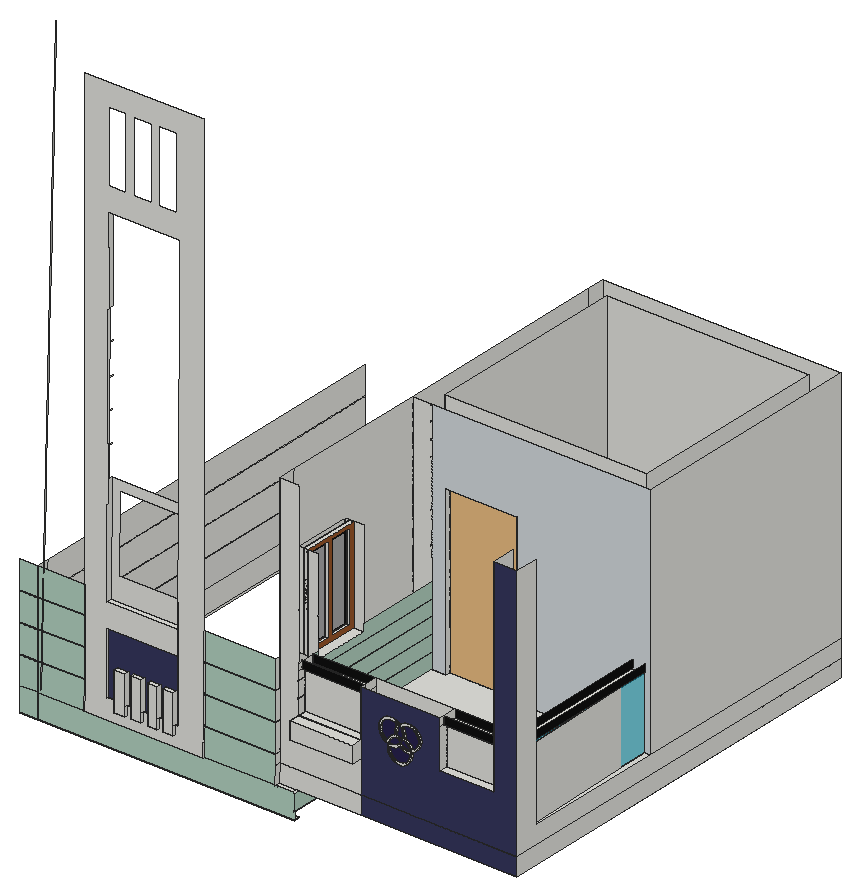
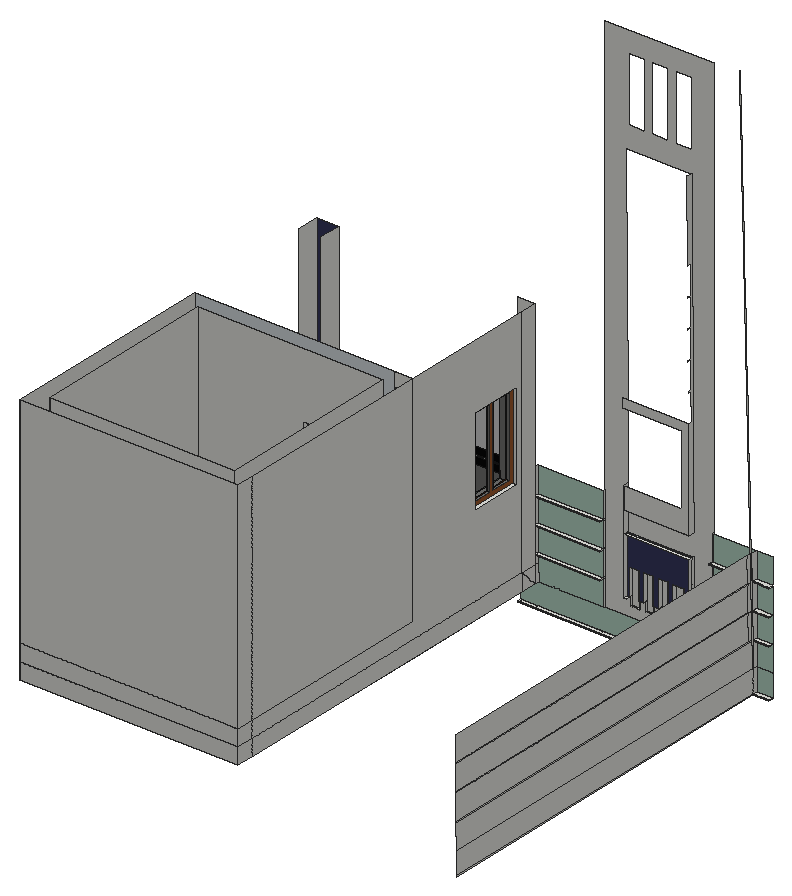
# SketchUp Ruby script. Lengths in inches.
U = 1.inch
M = Sketchup.active_model
def pt(a) = Geom::Point3d.new(a.map { |v| v * U })
def face(e, loops, mat)
  f = e.add_face(loops[0].map { |a| pt(a) })
  loops[1..].each { |l| e.add_face(l.map { |a| pt(a) }).erase! }
  f.material = f.back_material = mat if mat
  f
end
# faces: each face lists its corners as indices into pts; further lists are holes
def faces(e, pts, list, mat = nil) = list.each { |f| face(e, (f[0].is_a?(Array) ? f : [f]).map { |l| l.map { |i| pts[i] } }, mat) }
# xy, xz, yz: faces in a plane at the given z, y or x. An outline is a flat list of corners, or four numbers for a rectangle; further outlines are holes
def ring(l) = l.size == 4 ? [[l[0], l[1]], [l[2], l[1]], [l[2], l[3]], [l[0], l[3]]] : l.each_slice(2).to_a
def flat(e, list, mat, &to3) = list.each { |f| face(e, (f[0].is_a?(Array) ? f : [f]).map { |l| ring(l).map { |u, v| to3.(u, v) } }, mat) }
def xy(e, z, list, mat = nil) = flat(e, list, mat) { |x, y| [x, y, z] }
def xz(e, y, list, mat = nil) = flat(e, list, mat) { |x, z| [x, y, z] }
def yz(e, x, list, mat = nil) = flat(e, list, mat) { |y, z| [x, y, z] }
def lines(e, pts, list) = list.each { |a, b| e.add_line(pt(pts[a]), pt(pts[b])) }
# prism: a flat outline (further loops are holes) pulled along v
def prism(e, loops, v, mat = nil)
  f = face(e, loops, mat); d = Geom::Vector3d.new(v.map { |x| x * U })
  f.pushpull(f.normal.samedirection?(d) ? d.length : -d.length)
end
def box(e, o, s, mat = nil) = prism(e, [[o, [o[0] + s[0], o[1], o[2]], [o[0] + s[0], o[1] + s[1], o[2]], [o[0], o[1] + s[1], o[2]]]], [0, 0, s[2]], mat)
def at(x, y, z, deg = 0) = Geom::Transformation.translation(pt([x, y, z])) * Geom::Transformation.rotation(ORIGIN, Z_AXIS, deg.degrees)
def axes(o, x, y, z) = Geom::Transformation.new([*x, 0, *y, 0, *z, 0, *pt(o).to_a, 1])
def part(name) = M.definitions.add(name)
# library, detail: a bought-in or finely detailed component or shape, given as its bounding box
def library(name, o, s) = part(name).tap { |d| box(d.entities, o, s) }
def detail(e, o, s) = box(e.add_group.entities, o, s)
def put(e, d, t, mat = nil) = e.add_instance(d, t).tap { |i| i.material = mat if mat }
def group(e, t, mat = nil) = e.add_group.tap { |g| g.transformation = t; g.material = mat if mat }.entities
root = M.entities
M.materials.add("0235 AP 9121 dancing pink").color = [178, 209, 192]
M.materials.add("0328 AP 7205 PURPLE CHIFFON").color = [54, 55, 93]
M.materials.add("[0109_DarkSlateBlue]").color = [40, 34, 77]
M.materials.add("[0137_Black]").color = [17, 17, 17]
M.materials.add("[Square Glass Tile 01]").color = [212, 218, 221]
M.materials.add("[Translucent Glass Blue]").color = [0, 0, 0]
M.materials["[Translucent Glass Blue]"].alpha = 0.5
M.materials.add("[Translucent Glass Tinted]").color = [8, 201, 241]
M.materials["[Translucent Glass Tinted]"].alpha = 0.48
M.materials.add("[Wood Cherry Original]").color = [152, 86, 42]
c1 = library("doors",[0,-6.0625,0],[107.75,14.5625,198.25])
c2 = part("Glass Door - Open Shower")
box(c2.entities,[0,0,0.95],[40,1.5,72])
c3 = part("Group\#4")
xy(c3.entities,0,[[0,0,2,29]])
xy(c3.entities,2,[[0,2,2,13.5],[0,15.5,2,27]])
xy(c3.entities,46,[[0,2,2,13.5],[0,15.5,2,27]])
xy(c3.entities,48,[[0,0,2,29]])
xz(c3.entities,0,[[0,0,2,48]],"[Wood Cherry Original]")
xz(c3.entities,2,[[0,2,2,46]])
xz(c3.entities,13.5,[[0,2,2,46]])
xz(c3.entities,15.5,[[0,2,2,46]])
xz(c3.entities,27,[[0,2,2,46]])
xz(c3.entities,29,[[0,0,2,48]])
yz(c3.entities,0,[[2,2,13.5,46],[15.5,2,27,46]],"[Translucent Glass Blue]")
yz(c3.entities,0,[[[0,0,29,48],[2,2,13.5,46],[15.5,2,27,46]]],"[Wood Cherry Original]")
yz(c3.entities,2,[[[0,0,29,48],[2,2,13.5,46],[15.5,2,27,46]]],"[Wood Cherry Original]")
xy(root,107.5,[[48,70,56.72,72.5],[56.72,70,57,72.5],[57,70,186.5,72.5]])
xy(root,108,[[48,70,56.72,72.5],[57,70,80.72,72.5],[80.72,70,140.72,72.5],[140.72,70,176.72,72.5],[176.72,70,185.72,72.5],
  [185.72,70,186.5,72.5]])
xy(root,111.5,[[186,70,186.5,156.5]])
xy(root,112,[[186,70,186.5,156.5]])
xy(root,119.5,[[186,70,186.5,156.5]])
xy(root,120,[[80.6875,69.5,140.6875,70],[176.6875,70,185.6875,72.5],[176.6875,72.5,177,81.5,177,156.5,186,156.5,185.6875,72.5],[185.6875,72.5,186,156.5,297,156.5,297,84.5,285,84.5,285,72.5],[285,72.5,297,72.75],
  [285,72.75,297,84.5],[[177,156.5,297,276.5],[186,165.5,288,267.5]]])
xy(root,125.52,[[96.68,68.5,102.3,69.5],[105.23,68.5,110.3125,69.5],[113.75,68.5,118.42,69.5],[121.29,68.5,126.5,69.5]])
xy(root,129,[[177,72.5,297,81.5],[177,81.5,177,276.5,297,276.5,297,81.5,288,81.5,288,267.5,186,267.5,186,81.5],[186,81.5,288,267.5]])
xy(root,130.125,[[92,69.5,96.68,70.5],[102.3,69.5,105.23,70.5],[110.3125,69.5,113.75,70.5],[118.42,69.5,121.29,70.5],[126.5,69.5,128,70.5],
  [92,70.5,96.68,72.5],[126.5,70.5,128,72.5]])
xy(root,133.95,[[48,70,57,72.5],[57,70,81,72.5],[141,70,177,72.5]])
xy(root,134.45,[[48,70,57,72.5],[57,70,81,72.5],[141,70,177,72.5]])
xy(root,138,[[186.5,81.5,285,81.5,285,84.5,294.1875,84.5,294.1875,156.5,229.71,156.5,229.71,165.5,193.71,165.5,193.71,156.5,186.5,156.5],[294.1875,84.5,297,156.5],[177,156.5,177,276.5,297,276.5,297,156.5,229.71,156.5,229.71,165.5,288,165.5,288,267.5,186,267.5,186,165.5,193.71,165.5,193.71,156.5]])
xy(root,144.96,[[96.68,68.5,102.3,70.5],[105.23,68.5,110.3125,70.5],[113.75,68.5,118.42,70.5],[121.29,68.5,126.5,70.5]])
xy(root,145.5,[[186.5,66.9375,218.25,72.5],[186,72.5,186.5,156.5]])
xy(root,146,[[186,72.5,186.5,156.5]])
xy(root,148.39,[[48,70,57,72.5],[57,70,81,72.5],[141,70,177,72.5]])
xy(root,148.89,[[48,70,57,72.5],[57,70,81,72.5],[141,70,177,72.5]])
xy(root,153.5,[[186,72.5,186.5,156.5]])
xy(root,154,[[186.5,66.9375,218.25,72.5],[186,72.5,186.5,156.5],[186.5,72.5,218.25,77],[258.04,72.5,285,81.5],[186.5,77,218.25,81.5]])
xy(root,161.5,[[92,69.5,128,70.5],[92,70.5,128,72.5],[186,72.5,186.5,156.5]])
xy(root,162,[[186,72.5,186.5,156.5]])
xy(root,162.84,[[48,70,57,72.5],[57,70,81,72.5],[141,70,177,72.5]])
xy(root,163.34,[[48,70,57,72.5],[57,70,81,72.5],[141,70,177,72.5]])
xy(root,169.5,[[186,72.5,186.5,156.5]])
xy(root,170,[[186,72.5,186.5,156.5]])
xy(root,173.5,[[92,69.5,128,72.5]])
xy(root,174,[[258.04,74.75,285,81.5],[177,84.5,186.5,113.5],[288,84.5,294.1875,161.25]])
xy(root,174.01,[[186.5,74.625,218.25,77],[186.5,77,218.25,81.5]])
xz(root,66.9375,[[186.5,145.5,218.25,154]])
xz(root,68.5,[[96.68,125.52,102.3,144.96],[105.23,125.52,110.3125,144.96],[113.75,125.52,118.42,144.96],[121.29,125.52,126.5,144.96]])
xz(root,69.5,[[[80.6875,120,140.6875,120,141,133.95,141,408.9375,81,408.9375,81,133.95],[96.68,125.52,96.68,130.125,92,130.125,92,161.5,128,161.5,128,173.5,92,173.5,93,350.3125,129,350.3125,128.28,223.8125,128.07,185.5,128,173.5,128,130.125,126.5,130.125,126.5,125.52,121.29,125.52,121.29,130.125,118.42,130.125,118.42,125.52,113.75,125.52,113.75,130.125,110.3125,130.125,110.3125,125.52,105.23,125.52,105.23,130.125,102.3,130.125,102.3,125.52],[118.5625,362.07,127.375,397.89],[93,362.07,101.8125,397.89],[106,362.07,114.8125,397.89]]])
xz(root,70,[[48,108,56.72,108,56.6875,120,48,120],[57,108,186.5,108,186.5,111.5,186,111.5,186,112,186.5,112,186.5,119.5,186,119.5,185.6875,120,57,120],[48,120,56.6875,120,57,133.95,48,133.95],[57,120,80.6875,120,81,133.95,57,133.95],[140.6875,120,176.6875,120,177,129,177,133.95,141,133.95],
  [48,134.45,57,148.39],[57,134.45,81,148.39],[141,134.45,177,148.39],[48,148.89,57,162.84],[57,148.89,81,162.84],
  [141,148.89,177,162.84],[48,163.34,57,177.29],[57,163.34,81,177.29],[141,163.34,177,177.29]],"0235 AP 9121 dancing pink")
xz(root,70.5,[[92,130.125,96.68,130.125,96.68,144.96,102.3,144.96,102.3,130.125,105.23,130.125,105.23,144.96,110.3125,144.96,110.3125,130.125,113.75,130.125,113.75,144.96,118.42,144.96,118.42,130.125,121.29,130.125,121.29,144.96,126.5,144.96,126.5,130.125,128,130.125,128,161.5,92,161.5]],"0328 AP 7205 PURPLE CHIFFON")
xz(root,72,[[[238.6875,149.83,240.24,150.23,241.63,151.01,242.78,152.125,243.6,153.5,244.03,155.04,244.05,156.64,243.77,157.73,243.24,157.6,241.64,157.62,240.1,158.05,238.73,158.87,238.03,159.59,237.18,158.77,235.79,157.99,234.24,157.6,232.64,157.62,232.18,157.75,231.91,156.8,231.89,155.2,232.28,153.65,233.06,152.25,233.47,151.83,234.18,151.11,235.55,150.29,237.09,149.86],[238.57,150.84,237.23,150.85,235.95,151.22,234.8,151.9,234.19,152.53,233.87,152.86,233.22,154.02,232.89,155.32,232.9,156.62,234.36,156.6,236.16,157.06,237.79,157.96,238.01,158.18,238.1,158.08,239.7,157.13,241.49,156.62,243.03,156.6,243.05,156.52,243.03,155.18,242.67,153.9,241.99,152.75,241.03,151.82,239.86,151.16]],[[243.77,157.73,244.79,157.99,246.18,158.77,247.33,159.89,248.15,161.26,248.58,162.8,248.6,164.4,248.21,165.95,247.43,167.35,246.3125,168.49,244.9375,169.31,243.4,169.74,241.8,169.76,240.25,169.37,238.86,168.59,238.01,167.77,238.43,167.35,239.21,165.95,239.6,164.4,239.58,162.8,239.3125,161.85,240.39,161.54,241.76,160.73,242.88,159.58,243.66,158.1875],[244.39,158.92,243.69,160.18,242.39,161.52,240.79,162.47,240.55,162.54,240.58,162.66,240.6,164.52,240.15,166.32,239.375,167.7,239.46,167.78,240.625,168.43,241.92,168.76,243.26,168.75,244.54,168.38,245.6875,167.7,246.62,166.74,247.27,165.58,247.6,164.28,247.58,162.95,247.22,161.66,246.54,160.51,245.58,159.58]],[[232.18,157.75,232.34,158.34,233.16,159.71,233.46,160.01,234.3,160.83,235.7,161.61,236.72,161.86,236.4375,162.96,236.46,164.5625,236.89,166.1,237.71,167.48,238.01,167.77,237.3125,168.49,235.9375,169.31,234.4,169.74,232.8,169.76,231.25,169.37,229.86,168.59,228.71,167.48,227.89,166.1,227.46,164.5625,227.4375,162.96,227.83,161.41,228.61,160.02,229.73,158.87,231.1,158.05],[231.55,158.95,230.35,159.66,229.42,160.62,228.77,161.79,228.4375,163.08,228.46,164.42,228.82,165.7,229.5,166.85,230.46,167.78,231.625,168.43,232.92,168.76,234.26,168.75,235.54,168.38,236.68,167.7,235.97,166.5,235.46,164.71,235.44,162.85,235.5,162.59,235.33,162.54,233.7,161.63,232.77,160.72,232.37,160.34]]])
xz(root,72.5,[[56.72,107.5,57,108],[56.72,108,57,108,57,120,56.6875,120],[56.6875,120,57,120,57,133.95],[176.6875,120,218.25,120,218.25,129,177,129],[177,129,218.25,129,218.25,145.5,186,145.5,186,146,186.5,146,186.5,153.5,186,153.5,186,154,186.5,154,186.5,161.5,186,161.5,186,162,186.5,162,186.5,169.5,186,169.5,186,170,186.5,170,186.5,177.5,186,177.5,186,178,186.5,178,186.5,185.5,186,185.5,186,186,186.5,186,186.5,193.5,186,193.5,186,194,186.5,194,186.5,201.5,186,201.5,186,202,186.5,202,186.5,209.5,186,209.5,186,210,186.5,210,186.5,217.5,186,217.5,186,218,186.5,218,186.5,225.5,186,225.5,186,226,186.5,226,186.5,233.5,186,233.5,186,234,186.5,234,186.5,241.5,186,241.5,186,242,186.5,242,186.5,249.5,186,249.5,186,250,186.5,250,186.5,257.5,186,257.5,186,258,177,258],
  [186,145.5,218.25,145.5,218.25,154,186,154,186,153.5,186.5,153.5,186.5,146,186,146],[186,161.5,186.5,162],[186,169.5,186.5,170],[92,173.5,128,173.5,128.07,185.5,96.07,185.5,96.28,223.8125,128.28,223.8125,128.3125,228.63,92.3125,228.63]])
xz(root,72.5,[[218.25,120,297,129],[[218.25,129,297,129,297,258,285,258,285,154,258.04,154,258.04,178,218.25,178],[238.6875,149.83,237.09,149.86,235.55,150.29,234.18,151.11,233.47,151.83,233.06,152.25,232.28,153.65,231.89,155.2,231.91,156.8,232.18,157.75,231.1,158.05,229.73,158.87,228.61,160.02,227.83,161.41,227.4375,162.96,227.46,164.5625,227.89,166.1,228.71,167.48,229.86,168.59,231.25,169.37,232.8,169.76,234.4,169.74,235.9375,169.31,237.3125,168.49,238.01,167.77,238.86,168.59,240.25,169.37,241.8,169.76,243.4,169.74,244.9375,169.31,246.3125,168.49,247.43,167.35,248.21,165.95,248.6,164.4,248.58,162.8,248.15,161.26,247.33,159.89,246.18,158.77,244.79,157.99,243.77,157.73,244.05,156.64,244.03,155.04,243.6,153.5,242.78,152.125,241.63,151.01,240.24,150.23],[234.24,157.6,232.64,157.62,232.18,157.75,232.34,158.34,233.16,159.71,233.46,160.01,234.3,160.83,235.7,161.61,236.72,161.86,236.83,161.41,237.61,160.02,238.03,159.59,237.18,158.77,235.79,157.99],[243.24,157.6,241.64,157.62,240.1,158.05,238.73,158.87,238.03,159.59,238.33,159.89,239.15,161.26,239.3125,161.85,240.39,161.54,241.76,160.73,242.88,159.58,243.66,158.1875,243.77,157.73],[239.3125,161.85,238.85,161.98,237.25,162,236.72,161.86,236.4375,162.96,236.46,164.5625,236.89,166.1,237.71,167.48,238.01,167.77,238.43,167.35,239.21,165.95,239.6,164.4,239.58,162.8]]],"0328 AP 7205 PURPLE CHIFFON")
xz(root,72.5,[[238.57,150.84,239.86,151.16,241.03,151.82,241.99,152.75,242.67,153.9,243.03,155.18,243.05,156.52,243.03,156.6,241.49,156.62,239.7,157.13,238.1,158.08,238.01,158.18,237.79,157.96,236.16,157.06,234.36,156.6,232.9,156.62,232.89,155.32,233.22,154.02,233.87,152.86,234.19,152.53,234.8,151.9,235.95,151.22,237.23,150.85],[234.24,157.6,235.79,157.99,237.18,158.77,238.03,159.59,237.61,160.02,236.83,161.41,236.72,161.86,235.7,161.61,234.3,160.83,233.46,160.01,233.16,159.71,232.34,158.34,232.18,157.75,232.64,157.62],[243.24,157.6,243.77,157.73,243.66,158.1875,242.88,159.58,241.76,160.73,240.39,161.54,239.3125,161.85,239.15,161.26,238.33,159.89,238.03,159.59,238.73,158.87,240.1,158.05,241.64,157.62],[244.39,158.92,245.58,159.58,246.54,160.51,247.22,161.66,247.58,162.95,247.6,164.28,247.27,165.58,246.62,166.74,245.6875,167.7,244.54,168.38,243.26,168.75,241.92,168.76,240.625,168.43,239.46,167.78,239.375,167.7,240.15,166.32,240.6,164.52,240.58,162.66,240.55,162.54,240.79,162.47,242.39,161.52,243.69,160.18],[231.55,158.95,232.37,160.34,232.77,160.72,233.7,161.63,235.33,162.54,235.5,162.59,235.44,162.85,235.46,164.71,235.97,166.5,236.68,167.7,235.54,168.38,234.26,168.75,232.92,168.76,231.625,168.43,230.46,167.78,229.5,166.85,228.82,165.7,228.46,164.42,228.4375,163.08,228.77,161.79,229.42,160.62,230.35,159.66],
  [238.03,159.59,238.33,159.89,239.15,161.26,239.3125,161.85,238.85,161.98,237.25,162,236.72,161.86,236.83,161.41,237.61,160.02],[239.3125,161.85,239.58,162.8,239.6,164.4,239.21,165.95,238.43,167.35,238.01,167.77,237.71,167.48,236.89,166.1,236.46,164.5625,236.4375,162.96,236.72,161.86,237.25,162,238.85,161.98]],"[0109_DarkSlateBlue]")
xz(root,72.5,[[48,107.5,56.72,108],[57,107.5,186.5,108],[48,133.95,57,134.45],[57,133.95,81,134.45],[141,133.95,177,134.45],
  [48,148.39,57,148.89],[57,148.39,81,148.89],[141,148.39,177,148.89],[48,162.84,57,163.34],[57,162.84,81,163.34],
  [141,162.84,177,163.34]],"[0137_Black]")
xz(root,74.625,[[186.5,174.01,218.25,178]],"[0137_Black]")
xz(root,74.75,[[258.04,174,285,178]],"[0137_Black]")
xz(root,81.5,[[186.5,138,186.5,154,218.25,154,218.25,178,258.04,178,258.04,154,285,154,285,138]])
xz(root,81.5,[[258.04,174,285,178],[186.5,174.01,218.25,178]],"[0137_Black]")
xz(root,84.5,[[285,138,285,178,288,178,288,174,294.1875,174,294.1875,138],[294.1875,138,297,174],[177,174,177,222,186.5,222,186.5,218,186,218,186,217.5,186.5,217.5,186.5,210,186,210,186,209.5,186.5,209.5,186.5,202,186,202,186,201.5,186.5,201.5,186.5,194,186,194,186,193.5,186.5,193.5,186.5,186,186,186,186,185.5,186.5,185.5,186.5,178,186,178,186,177.5,186.5,177.5,186.5,174],[294.1875,174,297,178]])
xz(root,113.5,[[177,174,186.5,174,186.5,177.5,186,177.5,186,178,186.5,178,186.5,185.5,186,185.5,186,186,186.5,186,186.5,193.5,186,193.5,186,194,186.5,194,186.5,201.5,186,201.5,186,202,186.5,202,186.5,209.5,186,209.5,186,210,186.5,210,186.5,217.5,186,217.5,186,218,186.5,218,186.5,222,177,222]])
xz(root,156.5,[[177,138,186.5,138,186.5,145.5,186,145.5,186,146,186.5,146,186.5,153.5,186,153.5,186,154,186.5,154,186.5,161.5,186,161.5,186,162,186.5,162,186.5,169.5,186,169.5,186,170,186.5,170,186.5,177.5,186,177.5,186,178,186.5,178,186.5,185.5,186,185.5,186,186,186.5,186,186.5,193.5,186,193.5,186,194,186.5,194,186.5,201.5,186,201.5,186,202,186.5,202,186.5,209.5,186,209.5,186,210,186.5,210,186.5,217.5,186,217.5,186,218,186.5,218,186.5,225.5,186,225.5,186,226,186.5,226,186.5,233.5,186,233.5,186,234,186.5,234,186.5,241.5,186,241.5,186,242,186.5,242,186.5,249.5,186,249.5,186,250,186.5,250,186.5,257.5,186,257.5,186,258,177,258]])
xz(root,156.5,[[186.5,138,193.71,138,193.71,222,229.71,222,229.71,138,297,138,297,258,186,258,186,257.5,186.5,257.5,186.5,250,186,250,186,249.5,186.5,249.5,186.5,242,186,242,186,241.5,186.5,241.5,186.5,234,186,234,186,233.5,186.5,233.5,186.5,226,186,226,186,225.5,186.5,225.5,186.5,218,186,218,186,217.5,186.5,217.5,186.5,210,186,210,186,209.5,186.5,209.5,186.5,202,186,202,186,201.5,186.5,201.5,186.5,194,186,194,186,193.5,186.5,193.5,186.5,186,186,186,186,185.5,186.5,185.5,186.5,178,186,178,186,177.5,186.5,177.5,186.5,170,186,170,186,169.5,186.5,169.5,186.5,162,186,162,186,161.5,186.5,161.5,186.5,154,186,154,186,153.5,186.5,153.5,186.5,146,186,146,186,145.5,186.5,145.5]],"[Square Glass Tile 01]")
xz(root,161.25,[[288,174,294.1875,178]])
xz(root,165.5,[[186,138,186,258,288,258,288,138,229.71,138,229.71,222,193.71,222,193.71,138]])
xz(root,267.5,[[186,138,288,258]])
xz(root,276.5,[[177,120,297,129],[177,129,297,138],[177,138,297,258]])
yz(root,56.72,[[72.5,107.5,276.5,108]])
yz(root,57,[[70,108,72.5,120],[70,120,72.5,133.95],[72.5,133.95,72.5,134.45,72.52,134.45],[72.5,133.95,75.38,133.95,75.39,134.45,72.52,134.45],[75.38,133.95,75.39,134.45,276.5,134.45,276.5,133.95],
  [70,134.45,70,148.39,72.96,148.39,72.52,134.45],[72.52,134.45,75.39,134.45,75.6875,148.39,72.96,148.39],[75.39,134.45,75.6875,148.39,276.5,148.39,276.5,134.45],[72.5,148.39,72.5,148.89,72.97,148.89,72.96,148.39],[72.96,148.39,75.6875,148.39,75.7,148.89,72.97,148.89],
  [75.6875,148.39,75.7,148.89,276.5,148.89,276.5,148.39],[70,148.89,70,162.84,73.41,162.84,72.97,148.89],[72.97,148.89,75.7,148.89,76,162.84,73.41,162.84],[75.7,148.89,76,162.84,276.5,162.84,276.5,148.89],[72.5,162.84,72.5,163.34,73.43,163.34,73.41,162.84],
  [73.41,162.84,76,162.84,76.01,163.34,73.43,163.34],[76,162.84,76.01,163.34,276.5,163.34,276.5,162.84],[70,163.34,70,177.29,73.87,177.29,73.43,163.34],[73.43,163.34,76.01,163.34,76.31,177.29,73.87,177.29],[76.01,163.34,76.31,177.29,276.5,177.29,276.5,163.34]])
yz(root,81,[[69.5,133.95,72.5,134.45],[69.5,134.45,70,148.39],[69.5,148.39,72.5,148.89],[69.5,148.89,70,162.84],[69.5,162.84,72.5,163.34],
  [69.5,163.34,70,177.29]])
yz(root,92,[[69.5,130.125,70.5,161.5],[70.5,130.125,72.5,161.5]])
yz(root,96.68,[[68.5,125.52,69.5,130.125],[68.5,130.125,70.5,144.96]])
yz(root,102.3,[[68.5,125.52,69.5,130.125],[68.5,130.125,70.5,144.96]])
yz(root,105.23,[[68.5,125.52,69.5,130.125],[68.5,130.125,70.5,144.96]])
yz(root,110.3125,[[68.5,125.52,69.5,130.125],[68.5,130.125,70.5,144.96]])
yz(root,113.75,[[68.5,125.52,69.5,130.125],[68.5,130.125,70.5,144.96]])
yz(root,118.42,[[68.5,125.52,69.5,130.125],[68.5,130.125,70.5,144.96]])
yz(root,121.29,[[68.5,125.52,69.5,130.125],[68.5,130.125,70.5,144.96]])
yz(root,126.5,[[68.5,125.52,69.5,130.125],[68.5,130.125,70.5,144.96]])
yz(root,128,[[69.5,130.125,70.5,161.5],[70.5,130.125,72.5,161.5],[69.5,161.5,72.5,173.5]])
yz(root,141,[[69.5,133.95,72.5,134.45],[69.5,134.45,70,148.39],[69.5,148.39,72.5,148.89],[69.5,148.89,70,162.84],[69.5,162.84,72.5,163.34],
  [69.5,163.34,70,177.29]])
yz(root,177,[[81.5,120,267.22,129],[267.22,120,276.5,129],[70,129,72.5,133.95],[72.5,129,81.5,258],[[81.5,129,81.5,258,156.5,258,156.5,138,267.22,138,267.22,129],[84.5,174,113.5,222]],
  [267.22,129,276.5,138],[70,134.45,72.5,148.39],[156.5,138,267.22,258],[267.22,138,276.5,258],[70,148.89,72.5,162.84],
  [70,163.34,72.5,177.29]])
yz(root,186,[[70,111.5,156.5,112],[165.5,138,267.5,258],[72.5,145.5,156.5,146],[72.5,153.5,156.5,154],[72.5,161.5,156.5,162],
  [72.5,169.5,156.5,170]])
yz(root,186.5,[[66.9375,145.5,81.5,146],[66.9375,146,72.5,153.5],[72.5,146,81.5,153.5],[66.9375,153.5,81.5,154],[72.5,154,77,161.5],
  [72.5,162,77,169.5],[72.5,170,77,174.01],[72.5,174.01,74.625,177.5],[74.625,174.01,81.5,177.5]])
yz(root,186.5,[[70,112,156.5,119.5],[81.5,138,156.5,145.5],[81.5,146,156.5,153.5],[77,154,156.5,161.5],[77,162,156.5,169.5],
  [77,170,156.5,170,156.5,177.5,113.5,177.5,113.5,174,84.5,174,84.5,177.5,81.5,177.5,81.5,174.01,77,174.01]],"0235 AP 9121 dancing pink")
yz(root,193.71,[[156.5,138,165.5,222]])
yz(root,218.25,[[66.9375,145.5,72.5,154],[72.5,154,77,174.01],[77,154,81.5,174.01],[72.5,174.01,74.625,178],[74.625,174.01,81.5,178]])
yz(root,229.71,[[156.5,138,165.5,222]])
yz(root,258.04,[[72.5,154,81.5,174],[72.5,174,74.75,178],[74.75,174,81.5,178]])
yz(root,285,[[81.5,138,81.5,154,72.5,154,72.5,174,81.5,174,81.5,178,72.5,178,72.5,258,84.5,258,84.5,138],[72.5,174,74.75,178],[74.75,174,81.5,178]])
yz(root,288,[[165.5,138,267.5,258]])
yz(root,288,[[84.5,174,161.25,178]],"[0137_Black]")
yz(root,294.1875,[[84.5,174,161.25,178]],"[0137_Black]")
yz(root,294.1875,[[84.5,138,156.5,174]],"[Translucent Glass Tinted]")
yz(root,297,[[72.5,120,276.5,129],[72.5,129,276.5,129,276.5,138,84.5,138,84.5,258,72.5,258],[156.5,138,276.5,258]])
p = [[56.72,72.5,108],[56.6875,72.5,120],[56.6875,70,120],[56.72,70,108],[56.72,276.5,108],[56.6875,276.5,120],
  [186,70,119.5],[186,156.5,119.5],[185.6875,72.5,120],[185.6875,70,120],[186,156.5,120],[81,69.5,133.95],
  [81,70,133.95],[80.6875,70,120],[80.6875,69.5,120],[140.6875,69.5,120],[140.6875,70,120],[141,70,133.95],
  [141,69.5,133.95],[57,72.5,133.95],[57,70,133.95],[176.6875,72.5,120],[177,72.5,129],[177,70,129],
  [176.6875,70,120],[57,72.52,134.45],[57,72.96,148.39],[57,72.97,148.89],[57,73.41,162.84],[57,73.43,163.34],
  [57,73.87,177.29],[57,73.88,177.79],[57,74.32,191.73],[57,74.34,192.23],[57,74.78,206.18],[57,74.8,206.68],
  [57,75.24,220.63],[57,75.25,221.13],[57,75.69,235.07],[57,75.71,235.57],[57,76.15,249.52],[57,76.17,250.02],
  [57,76.61,263.97],[57,76.62,264.47],[57,77.0625,278.42],[57,77.08,278.92],[57,77.52,292.86],[57,77.53,293.36],
  [57,77.97,307.31],[57,77.99,307.81],[57,78.43,321.76],[57,78.45,322.26],[57,78.89,336.2],[57,78.9,336.7],
  [57,79.34,350.65],[57,79.36,351.15],[57,79.8,365.1],[57,79.82,365.6],[57,80.26,379.54],[57,80.27,380.04],
  [57,80.71,393.99],[57,80.73,394.49],[57,81.18,408.9375],[57,81.22,409.9375],[57,81.5,418.9375],[57,276.5,133.95],
  [57,75.38,133.95],[177,81.5,129],[177,81.5,120],[237.09,72.5,149.86],[238.6875,72.5,149.83],[238.6875,72,149.83],
  [237.09,72,149.86],[240.24,72.5,150.23],[240.24,72,150.23],[235.55,72.5,150.29],[235.55,72,150.29],[241.63,72.5,151.01],
  [241.63,72,151.01],[234.18,72.5,151.11],[234.18,72,151.11],[238.57,72.5,150.84],[237.23,72.5,150.85],[237.23,72,150.85],
  [238.57,72,150.84],[239.86,72.5,151.16],[239.86,72,151.16],[235.95,72.5,151.22],[235.95,72,151.22],[242.78,72.5,152.125],
  [242.78,72,152.125],[233.47,72.5,151.83],[233.47,72,151.83],[234.8,72.5,151.9],[234.8,72,151.9],[241.03,72.5,151.82],
  [241.03,72,151.82],[233.06,72.5,152.25],[233.06,72,152.25],[241.99,72.5,152.75],[241.99,72,152.75],[234.19,72.5,152.53],
  [234.19,72,152.53],[243.6,72.5,153.5],[243.6,72,153.5],[232.28,72.5,153.65],[232.28,72,153.65],[233.87,72.5,152.86],
  [233.87,72,152.86],[242.67,72.5,153.9],[242.67,72,153.9],[233.22,72.5,154.02],[233.22,72,154.02],[244.03,72.5,155.04],
  [244.03,72,155.04],[231.89,72.5,155.2],[231.89,72,155.2],[243.03,72.5,155.18],[243.03,72,155.18],[232.89,72.5,155.32],
  [232.89,72,155.32],[244.05,72.5,156.64],[244.05,72,156.64],[231.91,72.5,156.8],[231.91,72,156.8],[243.05,72.5,156.52],
  [243.05,72,156.52],[232.9,72.5,156.62],[232.9,72,156.62],[243.03,72.5,156.6],[243.03,72,156.6],[234.36,72.5,156.6],
  [234.36,72,156.6],[236.16,72.5,157.06],[236.16,72,157.06],[239.7,72.5,157.13],[241.49,72.5,156.62],[241.49,72,156.62],
  [239.7,72,157.13],[243.77,72.5,157.73],[243.77,72,157.73],[232.18,72.5,157.75],[232.18,72,157.75],[237.79,72.5,157.96],
  [237.79,72,157.96],[238.1,72.5,158.08],[238.1,72,158.08],[232.64,72.5,157.62],[232.64,72,157.62],[234.24,72.5,157.6],
  [234.24,72,157.6],[235.79,72.5,157.99],[235.79,72,157.99],[241.64,72.5,157.62],[240.1,72.5,158.05],[240.1,72,158.05],
  [241.64,72,157.62],[243.24,72.5,157.6],[243.24,72,157.6],[243.66,72.5,158.1875],[243.66,72,158.1875],[244.79,72.5,157.99],
  [244.79,72,157.99],[231.1,72.5,158.05],[231.1,72,158.05],[232.34,72.5,158.34],[232.34,72,158.34],[237.18,72.5,158.77],
  [237.18,72,158.77],[238.01,72.5,158.18],[238.01,72,158.18],[246.18,72.5,158.77],[246.18,72,158.77],[229.73,72.5,158.87],
  [229.73,72,158.87],[238.73,72.5,158.87],[238.73,72,158.87],[242.88,72.5,159.58],[242.88,72,159.58],[233.16,72.5,159.71],
  [233.16,72,159.71],[238.03,72.5,159.59],[238.03,72,159.59],[247.33,72.5,159.89],[247.33,72,159.89],[228.61,72.5,160.02],
  [228.61,72,160.02],[244.39,72.5,158.92],[243.69,72.5,160.18],[243.69,72,160.18],[244.39,72,158.92],[245.58,72.5,159.58],
  [245.58,72,159.58],[231.55,72.5,158.95],[230.35,72.5,159.66],[230.35,72,159.66],[231.55,72,158.95],[232.37,72.5,160.34],
  [232.37,72,160.34],[241.76,72.5,160.73],[241.76,72,160.73],[246.54,72.5,160.51],[246.54,72,160.51],[229.42,72.5,160.62],
  [229.42,72,160.62],[233.46,72.5,160.01],[233.46,72,160.01],[248.15,72.5,161.26],[248.15,72,161.26],[227.83,72.5,161.41],
  [227.83,72,161.41],[234.3,72.5,160.83],[234.3,72,160.83],[242.39,72.5,161.52],[242.39,72,161.52],[232.77,72.5,160.72],
  [232.77,72,160.72],[247.22,72.5,161.66],[247.22,72,161.66],[228.77,72.5,161.79],[228.77,72,161.79],[233.7,72.5,161.63],
  [233.7,72,161.63],[240.39,72.5,161.54],[240.39,72,161.54],[235.7,72.5,161.61],[235.7,72,161.61],[248.58,72.5,162.8],
  [248.58,72,162.8],[227.4375,72.5,162.96],[227.4375,72,162.96],[239.3125,72.5,161.85],[239.3125,72,161.85],[240.79,72.5,162.47],
  [240.79,72,162.47],[235.33,72.5,162.54],[235.33,72,162.54],[236.72,72.5,161.86],[236.72,72,161.86],[247.58,72.5,162.95],
  [247.58,72,162.95],[228.4375,72.5,163.08],[228.4375,72,163.08],[239.58,72.5,162.8],[239.58,72,162.8],[236.4375,72.5,162.96],
  [236.4375,72,162.96],[235.5,72.5,162.59],[235.5,72,162.59],[240.55,72.5,162.54],[240.55,72,162.54],[240.58,72.5,162.66],
  [240.58,72,162.66],[235.44,72.5,162.85],[235.44,72,162.85],[240.6,72.5,164.52],[240.6,72,164.52],[235.46,72.5,164.71],
  [235.46,72,164.71],[239.6,72.5,164.4],[239.6,72,164.4],[248.6,72.5,164.4],[248.6,72,164.4],[247.6,72.5,164.28],
  [247.6,72,164.28],[227.46,72.5,164.5625],[227.46,72,164.5625],[236.46,72.5,164.5625],[236.46,72,164.5625],[228.46,72.5,164.42],
  [228.46,72,164.42],[247.27,72.5,165.58],[247.27,72,165.58],[228.82,72.5,165.7],[228.82,72,165.7],[239.21,72.5,165.95],
  [239.21,72,165.95],[248.21,72.5,165.95],[248.21,72,165.95],[240.15,72.5,166.32],[240.15,72,166.32],[227.89,72.5,166.1],
  [227.89,72,166.1],[236.89,72.5,166.1],[236.89,72,166.1],[235.97,72.5,166.5],[235.97,72,166.5],[246.62,72.5,166.74],
  [246.62,72,166.74],[229.5,72.5,166.85],[229.5,72,166.85],[238.43,72.5,167.35],[238.43,72,167.35],[247.43,72.5,167.35],
  [247.43,72,167.35],[228.71,72.5,167.48],[228.71,72,167.48],[237.71,72.5,167.48],[237.71,72,167.48],[239.375,72.5,167.7],
  [239.375,72,167.7],[236.68,72.5,167.7],[236.68,72,167.7],[245.6875,72.5,167.7],[245.6875,72,167.7],[230.46,72.5,167.78],
  [230.46,72,167.78],[238.01,72.5,167.77],[238.01,72,167.77],[246.3125,72.5,168.49],[246.3125,72,168.49],[229.86,72.5,168.59],
  [229.86,72,168.59],[235.54,72.5,168.38],[235.54,72,168.38],[239.46,72.5,167.78],[239.46,72,167.78],[244.54,72.5,168.38],
  [244.54,72,168.38],[231.625,72.5,168.43],[231.625,72,168.43],[237.3125,72.5,168.49],[237.3125,72,168.49],[238.86,72.5,168.59],
  [238.86,72,168.59],[240.625,72.5,168.43],[240.625,72,168.43],[232.92,72.5,168.76],[232.92,72,168.76],[234.26,72.5,168.75],
  [234.26,72,168.75],[241.92,72.5,168.76],[241.92,72,168.76],[243.26,72.5,168.75],[243.26,72,168.75],[235.9375,72.5,169.31],
  [235.9375,72,169.31],[244.9375,72.5,169.31],[244.9375,72,169.31],[231.25,72.5,169.37],[231.25,72,169.37],[240.25,72.5,169.37],
  [240.25,72,169.37],[234.4,72.5,169.74],[234.4,72,169.74],[243.4,72.5,169.74],[243.4,72,169.74],[232.8,72.5,169.76],
  [232.8,72,169.76],[241.8,72.5,169.76],[241.8,72,169.76],[92,72.5,173.5],[92.3125,72.5,228.63],[92.3125,70.5,228.63],
  [92.4,70.5,243.66],[92.4,72.5,243.66],[92.4,72.5,244.16],[92.4,70.5,244.16],[92.48,70.5,259.18],[92.48,72.5,259.18],
  [92.49,72.5,259.68],[92.49,70.5,259.68],[92.57,70.5,274.7],[92.57,72.5,274.7],[92.58,72.5,275.2],[92.58,70.5,275.2],
  [92.66,70.5,290.23],[92.66,72.5,290.23],[92.66,72.5,290.73],[92.66,70.5,290.73],[92.75,70.5,306.25],[92.75,72.5,306.25],
  [93,72.5,350.3125],[93,69.5,350.3125],[92,69.5,173.5],[128.07,72.5,185.5],[128,72.5,173.5],[128,69.5,173.5],
  [128.07,69.5,185.5],[186.5,77,162],[186.5,77,161.5],[186.5,77,170],[186.5,77,169.5]]
faces(root,p,[[0,1,2,3],[1,0,4,5],[6,7,8,9],[10,8,7],[11,12,13,14],[15,16,17,18],[1,19,20,2],[21,22,23,24],
  [1,19,25,26,27,28,29,30,31,32,33,34,35,36,37,38,39,40,41,42,43,44,45,46,47,48,49,50,51,52,53,54,55,56,57,58,59,60,61,62,63,64],[19,1,5,65,66],[22,67,21],[68,21,67],[69,70,71,72],[70,73,74,71],[75,69,72,76],[73,77,78,74],
  [79,75,76,80],[81,82,83,84],[85,81,84,86],[82,87,88,83],[77,89,90,78],[91,79,80,92],[87,93,94,88],[95,85,86,96],
  [97,91,92,98],[99,95,96,100],[93,101,102,94],[89,103,104,90],[105,97,98,106],[101,107,108,102],[109,99,100,110],[107,111,112,108],
  [103,113,114,104],[115,105,106,116],[117,109,110,118],[111,119,120,112],[113,121,122,114],[123,115,116,124],[125,117,118,126],[119,127,128,120],
  [129,125,126,130],[127,131,132,128],[131,133,134,132],[135,136,137,138],[136,129,130,137],[121,139,140,122],[141,123,124,142],[133,143,144,134],
  [145,135,138,146],[147,141,142,148],[149,147,148,150],[151,149,150,152],[153,154,155,156],[157,153,156,158],[139,157,158,140],[159,139,140,160],
  [139,161,162,140],[163,141,142,164],[141,165,166,142],[167,151,152,168],[143,169,170,144],[161,171,172,162],[173,163,164,174],[169,145,146,170],
  [154,175,176,155],[177,159,160,178],[165,179,180,166],[181,167,168,182],[171,183,184,172],[185,173,174,186],[175,181,182,176],[187,188,189,190],
  [191,187,190,192],[193,194,195,196],[197,193,196,198],[199,177,178,200],[201,191,192,202],[194,203,204,195],[179,205,206,180],[183,207,208,184],
  [209,185,186,210],[205,211,212,206],[188,213,214,189],[215,197,198,216],[217,201,202,218],[203,219,220,204],[221,215,216,222],[223,199,200,224],
  [211,225,226,212],[207,227,228,208],[229,209,210,230],[231,223,224,232],[213,233,234,214],[235,221,222,236],[225,237,238,226],[239,217,218,240],
  [219,241,242,220],[243,231,232,244],[237,245,246,238],[247,235,236,248],[233,249,250,234],[249,251,252,250],[253,247,248,254],[251,255,256,252],
  [257,253,254,258],[259,243,244,260],[227,261,262,228],[263,239,240,264],[265,229,230,266],[245,267,268,246],[241,269,270,242],[271,263,264,272],
  [269,273,274,270],[275,259,260,276],[261,277,278,262],[255,279,280,256],[281,265,266,282],[267,283,284,268],[285,257,258,286],[287,271,272,288],
  [273,289,290,274],[291,275,276,292],[277,293,294,278],[295,281,282,296],[283,297,298,284],[279,299,300,280],[301,285,286,302],[303,287,288,304],
  [289,305,306,290],[307,291,292,308],[293,309,310,294],[311,295,296,312],[297,307,308,298],[313,301,302,314],[299,315,316,300],[317,303,304,318],
  [305,319,320,306],[307,321,322,308],[323,307,308,324],[315,325,326,316],[319,327,328,320],[329,313,314,330],[325,331,332,326],[333,317,318,334],
  [321,335,336,322],[309,337,338,310],[339,311,312,340],[341,323,324,342],[327,329,330,328],[331,333,334,332],[335,343,344,336],[337,345,346,338],
  [347,339,340,348],[349,341,342,350],[343,347,348,344],[345,349,350,346],[351,352,353,354,355,356,357,358,359,360,361,362,363,364,365,366,367,368,369,370,371,372,373,374],[375,376,377,378]])
lines(root,p,[[379,380],[381,382]])
put(root,c1,axes([193.71,160.82,138],[0.33411,0,0],[0,0.3128,0],[0,0,0.42371]))
put(root,c2,axes([295.84,84.51,137.52],[-0.05229,1.80264,0],[-0.43539,-0.01263,0],[0,0,0.50091]))
put(root,c2,axes([258.04,77,153.74],[0.79375,0,0],[0,0.27223,0],[0,0,0.27223]))
put(root,c2,axes([186.5,76.79,153.87],[0.79375,0,0],[0,0.27223,0],[0,0,0.27223]))
put(root,c3,at(179.5,84.5,174))
